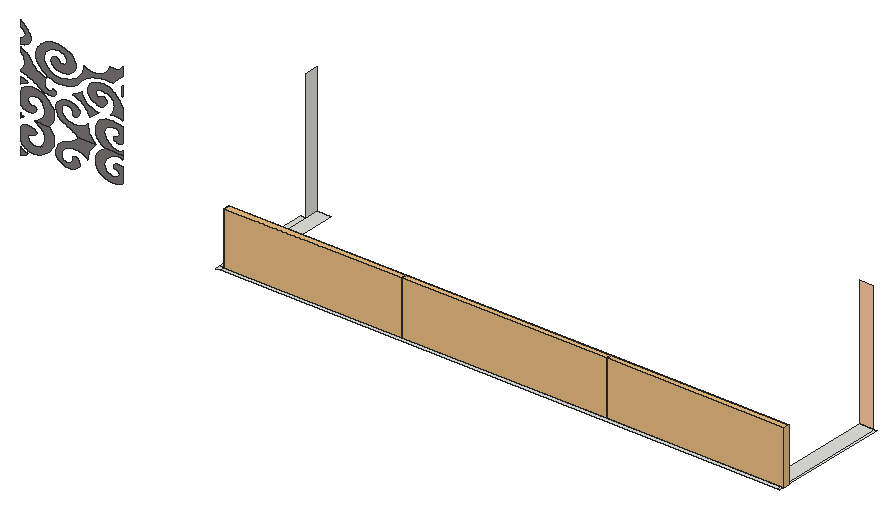
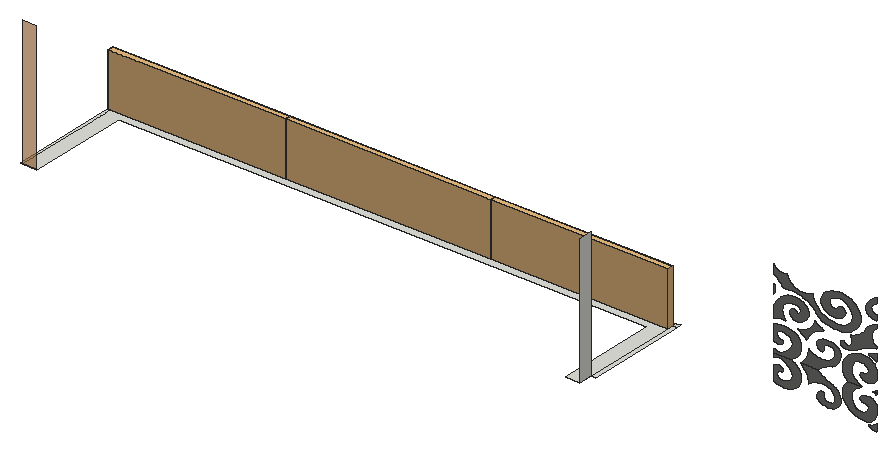
# SketchUp Ruby script. Lengths in inches.
U = 1.inch
M = Sketchup.active_model
def pt(a) = Geom::Point3d.new(a.map { |v| v * U })
def face(e, loops, mat)
  f = e.add_face(loops[0].map { |a| pt(a) })
  loops[1..].each { |l| e.add_face(l.map { |a| pt(a) }).erase! }
  f.material = f.back_material = mat if mat
  f
end
# faces: each face lists its corners as indices into pts; further lists are holes
def faces(e, pts, list, mat = nil) = list.each { |f| face(e, (f[0].is_a?(Array) ? f : [f]).map { |l| l.map { |i| pts[i] } }, mat) }
# xy, xz, yz: faces in a plane at the given z, y or x. An outline is a flat list of corners, or four numbers for a rectangle; further outlines are holes
def ring(l) = l.size == 4 ? [[l[0], l[1]], [l[2], l[1]], [l[2], l[3]], [l[0], l[3]]] : l.each_slice(2).to_a
def flat(e, list, mat, &to3) = list.each { |f| face(e, (f[0].is_a?(Array) ? f : [f]).map { |l| ring(l).map { |u, v| to3.(u, v) } }, mat) }
def xy(e, z, list, mat = nil) = flat(e, list, mat) { |x, y| [x, y, z] }
def xz(e, y, list, mat = nil) = flat(e, list, mat) { |x, z| [x, y, z] }
def yz(e, x, list, mat = nil) = flat(e, list, mat) { |y, z| [x, y, z] }
def lines(e, pts, list) = list.each { |a, b| e.add_line(pt(pts[a]), pt(pts[b])) }
# prism: a flat outline (further loops are holes) pulled along v
def prism(e, loops, v, mat = nil)
  f = face(e, loops, mat); d = Geom::Vector3d.new(v.map { |x| x * U })
  f.pushpull(f.normal.samedirection?(d) ? d.length : -d.length)
end
def box(e, o, s, mat = nil) = prism(e, [[o, [o[0] + s[0], o[1], o[2]], [o[0] + s[0], o[1] + s[1], o[2]], [o[0], o[1] + s[1], o[2]]]], [0, 0, s[2]], mat)
def at(x, y, z, deg = 0) = Geom::Transformation.translation(pt([x, y, z])) * Geom::Transformation.rotation(ORIGIN, Z_AXIS, deg.degrees)
def axes(o, x, y, z) = Geom::Transformation.new([*x, 0, *y, 0, *z, 0, *pt(o).to_a, 1])
def part(name) = M.definitions.add(name)
# library, detail: a bought-in or finely detailed component or shape, given as its bounding box
def library(name, o, s) = part(name).tap { |d| box(d.entities, o, s) }
def detail(e, o, s) = box(e.add_group.entities, o, s)
def put(e, d, t, mat = nil) = e.add_instance(d, t).tap { |i| i.material = mat if mat }
def group(e, t, mat = nil) = e.add_group.tap { |g| g.transformation = t; g.material = mat if mat }.entities
root = M.entities
M.materials.add("[0043_SaddleBrown]4").color = [124, 123, 122]
M.materials.add("[Granite Light Gray]").color = [149, 148, 144]
M.materials.add("[Wood Floor]").color = [224, 152, 88]
M.materials["[Wood Floor]"].alpha = 0.68
c1 = library("Glass Railing",[0,0,0],[139.5,4.76,42])
xy(root,293,[[1798.95,556.4375,1802.38,559.875],[1802.38,556.4375,2240.81,559.875],[2240.81,556.4375,2242.75,559.875],[1798.95,559.875,1802.38,640.11],[1802.38,559.875,2240.81,559.875,2240.81,651.03,2229.49,651.03,2229.49,571.2,1813.71,571.2,1813.71,651.03,1802.38,651.03],
  [2240.81,559.875,2242.75,651.03]])
xz(root,589.17,[[1618.6,295.77,1618.6,301,1618.96,300.64,1619.34,300.3,1619.76,299.98,1620.21,299.68,1620.6875,299.4,1621.1875,299.15,1621.71,298.92,1622.26,298.72,1622.82,298.54,1623.39,298.4,1623.98,298.28,1624.58,298.1875,1624.22,297.86,1623.82,297.54,1623.39,297.25,1622.9375,296.98,1622.46,296.74,1621.95,296.52,1621.43,296.32,1620.89,296.15,1620.33,296.02,1619.76,295.91,1619.18,295.82],[1656.57,299.46,1654.58,299.6,1652.66,300.03,1650.91,300.72,1649.39,301.66,1648.17,302.81,1647.3,304.1,1646.8,305.5,1646.66,306.54,1646.64,307.57,1646.74,308.61,1646.97,309.63,1647.32,310.64,1647.8,311.62,1648.39,312.57,1649.09,313.47,1649.9,314.33,1650.81,315.14,1651.81,315.88,1652.91,316.56,1654.06,316.875,1655.18,317.24,1656.28,317.65,1657.34,318.1,1658.37,318.59,1659.35,319.13,1660.3,319.7,1661.19,320.3125,1662.04,320.96,1662.84,321.64,1663.58,322.35,1664.27,323.09,1678.03,323.09,1677.05,322.2,1676.15,321.27,1675.33,320.31,1674.59,319.31,1673.93,318.28,1673.37,317.22,1672.9,316.14,1672.52,315.03,1672.24,313.92,1672.05,312.79,1671.96,311.66,1671.96,310.53,1671.38,311.07,1670.75,311.58,1670.07,312.0625,1669.34,312.51,1668.58,312.91,1667.77,313.28,1666.93,313.6,1666.0625,313.88,1665.17,314.11,1664.25,314.3,1663.32,314.44,1662.38,314.54,1660.75,314.5625,1659.14,314.41,1657.58,314.07,1656.12,313.56,1654.78,312.89,1653.61,312.07,1652.63,311.14,1651.87,310.1,1651.34,308.99,1651.06,307.84,1651.03,306.66,1651.27,305.5,1651.52,304.93,1651.91,304.41,1652.43,303.9375,1653.0625,303.54,1653.78,303.24,1654.5625,303.04,1655.38,302.93,1656.21,302.94,1657.03,303.06,1657.8,303.28,1658.51,303.6,1659.12,304,1659.28,304.24,1659.42,304.5,1659.55,304.75,1659.65,305.01,1659.73,305.28,1659.8,305.54,1659.84,305.8125,1659.86,306.08,1659.86,306.36,1659.84,306.625,1659.8,306.9,1659.74,307.16,1659.71,307.41,1659.73,307.66,1659.82,307.9,1659.96,308.13,1660.15,308.34,1660.39,308.52,1660.67,308.67,1660.98,308.78,1661.31,308.85,1661.65,308.875,1662,308.86,1662.33,308.8,1662.94,308.46,1663.49,308.07,1663.98,307.64,1664.4,307.17,1664.75,306.68,1665.02,306.15,1665.21,305.61,1665.32,305.0625,1665.34,304.51,1665.28,303.95,1665.14,303.41,1664.91,302.875,1663.71,301.72,1662.2,300.77,1660.46,300.06,1658.56,299.61],[1629.43,299.94,1627.86,299.97,1626.32,300.16,1624.83,300.52,1623.43,301.04,1622.16,301.7,1621.05,302.5,1620.12,303.41,1619.39,304.41,1618.88,305.48,1618.6,306.59,1618.6,314.54,1619.0625,315.41,1619.74,316.19,1620.61,316.875,1621.65,317.42,1622.81,317.82,1624.05,318.05,1625.33,318.11,1626.61,318,1627.83,317.71,1628.96,317.27,1629.94,316.67,1630.76,315.96,1631,315.64,1631.16,315.29,1631.23,314.93,1631.21,314.57,1631.09,314.22,1630.89,313.88,1630.61,313.58,1630.26,313.32,1629.85,313.11,1629.39,312.96,1628.91,312.86,1628.4,312.84,1627.74,312.8,1627.09,312.6875,1626.48,312.49,1625.93,312.23,1625.44,311.89,1625.05,311.51,1624.75,311.08,1624.56,310.62,1624.48,310.14,1624.52,309.66,1624.67,309.1875,1624.94,308.75,1625.32,307.98,1625.89,307.28,1626.64,306.67,1627.53,306.17,1628.53,305.8,1629.62,305.58,1630.74,305.5,1631.86,305.58,1632.95,305.81,1633.95,306.18,1635.37,307.48,1636.5,308.92,1637.31,310.46,1637.79,312.08,1637.91,313.73,1637.6875,315.38,1637.11,316.98,1636.21,318.5,1634.99,319.9,1633.49,321.15,1631.74,322.22,1629.79,323.09,1640.73,323.09,1642.56,321.23,1643.95,319.18,1644.89,317,1645.33,314.75,1645.27,312.47,1644.71,310.22,1643.67,308.07,1642.17,306.0625,1640.25,304.25,1637.96,302.68,1635.35,301.39,1632.49,300.42,1630.99,300.1],[1691.27,301.35,1688.56,301.57,1685.97,302.17,1683.6,303.12,1681.53,304.39,1679.84,305.93,1678.61,307.67,1677.88,309.5625,1677.68,311.52,1678.02,313.46,1678.1,314.46,1678.31,315.44,1678.63,316.41,1679.08,317.35,1679.65,318.26,1680.33,319.125,1681.12,319.94,1682.01,320.71,1682.99,321.41,1684.05,322.04,1685.19,322.6,1686.4,323.09,1698.99,323.09,1698.99,320.125,1698.69,320.4,1698.35,320.65,1697.96,320.87,1697.55,321.05,1697.11,321.2,1696.64,321.3,1696.17,321.37,1695.68,321.4,1695.19,321.38,1694.71,321.32,1694.25,321.23,1693.8,321.09,1692.72,320.67,1691.68,320.19,1690.7,319.66,1689.77,319.08,1688.9,318.45,1688.1,317.78,1687.37,317.07,1686.7,316.33,1686.12,315.55,1685.62,314.74,1685.19,313.91,1684.85,313.06,1684.66,312.23,1684.625,311.39,1684.77,310.55,1685.07,309.74,1685.54,308.97,1686.15,308.25,1686.9,307.61,1687.78,307.05,1688.76,306.59,1689.8125,306.24,1690.93,306,1692.09,305.875,1693.15,305.92,1694.17,306.14,1695.08,306.54,1695.83,307.09,1696.37,307.75,1696.67,308.49,1696.71,309.26,1696.49,310.01,1696.02,310.7,1695.33,311.28,1694.46,311.73,1693.47,312.01,1693.23,312,1692.98,312.01,1692.74,312.06,1692.52,312.13,1692.3125,312.23,1692.14,312.36,1691.99,312.5,1691.89,312.66,1691.82,312.83,1691.79,313.01,1691.81,313.18,1691.87,313.36,1692.15,313.84,1692.54,314.28,1693.03,314.67,1693.59,315,1694.22,315.25,1694.91,315.43,1695.62,315.53,1696.35,315.54,1697.0625,315.47,1697.76,315.3125,1698.4,315.08,1698.99,314.77,1698.99,302.99,1696.58,302.08,1693.98,301.53],[1618.6,321.36,1618.6,323.09,1621,323.09,1620.68,323.07,1620.38,323.03,1620.08,322.96,1619.8,322.86,1619.54,322.73,1619.3,322.58,1619.1,322.41,1618.92,322.22,1618.78,322.02,1618.68,321.81,1618.62,321.59],
  [1618.6,323.09,1621,323.09,1620.68,323.1,1620.38,323.15,1620.08,323.22,1619.8,323.32,1619.54,323.45,1619.3,323.59,1619.1,323.76,1618.92,323.95,1618.78,324.16,1618.68,324.37,1618.62,324.59,1618.6,324.82],[1629.79,323.09,1640.73,323.09,1642.56,324.95,1643.95,326.99,1644.89,329.17,1645.33,331.43,1645.27,333.71,1644.71,335.95,1643.67,338.11,1642.17,340.11,1640.25,341.93,1637.96,343.5,1635.35,344.78,1632.49,345.76,1630.99,346.08,1629.43,346.23,1627.86,346.21,1626.32,346.02,1624.83,345.66,1623.43,345.14,1622.16,344.47,1621.05,343.68,1620.12,342.77,1619.39,341.77,1618.88,340.7,1618.6,339.58,1618.6,331.63,1619.0625,330.77,1619.74,329.98,1620.61,329.3,1621.65,328.75,1622.81,328.36,1624.05,328.12,1625.33,328.0625,1626.61,328.18,1627.83,328.46,1628.96,328.91,1629.94,329.5,1630.76,330.22,1631,330.54,1631.16,330.88,1631.23,331.24,1631.21,331.61,1631.09,331.96,1630.89,332.29,1630.61,332.6,1630.26,332.86,1629.85,333.07,1629.39,333.22,1628.91,333.3125,1628.4,333.34,1627.74,333.375,1627.09,333.49,1626.48,333.68,1625.93,333.95,1625.44,334.28,1625.05,334.67,1624.75,335.1,1624.56,335.5625,1624.48,336.04,1624.52,336.52,1624.67,336.99,1624.94,337.43,1625.32,338.2,1625.89,338.9,1626.64,339.51,1627.53,340,1628.53,340.375,1629.62,340.6,1630.74,340.68,1631.86,340.6,1632.95,340.37,1633.95,340,1635.37,338.7,1636.5,337.26,1637.31,335.71,1637.79,334.1,1637.91,332.44,1637.6875,330.8,1637.11,329.2,1636.21,327.68,1634.99,326.28,1633.49,325.02,1631.74,323.95],[1664.27,323.09,1678.03,323.09,1677.05,323.97,1676.15,324.9,1675.33,325.87,1674.59,326.87,1673.93,327.9,1673.37,328.96,1672.9,330.04,1672.52,331.14,1672.24,332.26,1672.05,333.38,1671.96,334.51,1671.96,335.65,1671.38,335.11,1670.75,334.59,1670.07,334.11,1669.34,333.67,1668.58,333.27,1667.77,332.9,1666.93,332.58,1666.0625,332.3,1665.17,332.0625,1664.25,331.875,1663.32,331.73,1662.38,331.64,1660.75,331.61,1659.14,331.77,1657.58,332.11,1656.12,332.62,1654.78,333.29,1653.61,334.1,1652.63,335.04,1651.87,336.08,1651.34,337.18,1651.06,338.34,1651.03,339.51,1651.27,340.67,1651.52,341.24,1651.91,341.77,1652.43,342.24,1653.0625,342.63,1653.78,342.9375,1654.5625,343.14,1655.38,343.24,1656.21,343.23,1657.03,343.12,1657.8,342.9,1658.51,342.58,1659.12,342.18,1659.28,341.93,1659.42,341.68,1659.55,341.42,1659.65,341.16,1659.73,340.9,1659.8,340.63,1659.84,340.36,1659.86,340.09,1659.86,339.82,1659.84,339.55,1659.8,339.28,1659.74,339.01,1659.71,338.76,1659.73,338.52,1659.82,338.27,1659.96,338.05,1660.15,337.84,1660.39,337.66,1660.67,337.51,1660.98,337.4,1661.31,337.33,1661.65,337.3,1662,337.32,1662.33,337.37,1662.94,337.72,1663.49,338.11,1663.98,338.54,1664.4,339,1664.75,339.5,1665.02,340.02,1665.21,340.5625,1665.32,341.11,1665.34,341.67,1665.28,342.22,1665.14,342.77,1664.91,343.3,1663.71,344.45,1662.2,345.41,1660.46,346.12,1658.56,346.5625,1656.57,346.72,1654.58,346.58,1652.66,346.15,1650.91,345.45,1649.39,344.51,1648.17,343.37,1647.3,342.07,1646.8,340.67,1646.66,339.64,1646.64,338.6,1646.74,337.57,1646.97,336.54,1647.32,335.54,1647.8,334.56,1648.39,333.61,1649.09,332.7,1649.9,331.84,1650.81,331.04,1651.81,330.3,1652.91,329.62,1654.06,329.3,1655.18,328.9375,1656.28,328.53,1657.34,328.08,1658.37,327.58,1659.35,327.05,1660.3,326.47,1661.19,325.86,1662.04,325.22,1662.84,324.54,1663.58,323.83],[1686.4,323.09,1698.99,323.09,1698.99,326.05,1698.69,325.77,1698.35,325.53,1697.96,325.31,1697.55,325.125,1697.11,324.98,1696.64,324.87,1696.17,324.8,1695.68,324.78,1695.19,324.79,1694.71,324.85,1694.25,324.95,1693.8,325.09,1692.72,325.51,1691.68,325.99,1690.7,326.52,1689.77,327.1,1688.9,327.72,1688.1,328.39,1687.37,329.1,1686.7,329.85,1686.12,330.625,1685.62,331.43,1685.19,332.27,1684.85,333.12,1684.66,333.95,1684.625,334.79,1684.77,335.62,1685.07,336.44,1685.54,337.21,1686.15,337.92,1686.9,338.57,1687.78,339.125,1688.76,339.58,1689.8125,339.9375,1690.93,340.18,1692.09,340.3,1693.15,340.26,1694.17,340.03,1695.08,339.64,1695.83,339.09,1696.37,338.43,1696.67,337.6875,1696.71,336.92,1696.49,336.17,1696.02,335.48,1695.33,334.89,1694.46,334.45,1693.47,334.17,1693.23,334.18,1692.98,334.17,1692.74,334.12,1692.52,334.05,1692.3125,333.95,1692.14,333.82,1691.99,333.68,1691.89,333.52,1691.82,333.35,1691.79,333.17,1691.81,332.99,1691.87,332.82,1692.15,332.34,1692.54,331.9,1693.03,331.51,1693.59,331.18,1694.22,330.92,1694.91,330.74,1695.62,330.65,1696.35,330.64,1697.0625,330.71,1697.76,330.86,1698.4,331.1,1698.99,331.41,1698.99,343.1875,1696.58,344.1,1693.98,344.65,1691.27,344.82,1688.56,344.61,1685.97,344.01,1683.6,343.06,1681.53,341.79,1679.84,340.25,1678.61,338.5,1677.88,336.61,1677.68,334.66,1678.02,332.71,1678.1,331.72,1678.31,330.74,1678.63,329.77,1679.08,328.83,1679.65,327.92,1680.33,327.05,1681.12,326.23,1682.01,325.47,1682.99,324.77,1684.05,324.13,1685.19,323.57],[1673.16,341.21,1673.69,341.68,1674.23,342.15,1674.78,342.61,1675.34,343.0625,1675.91,343.51,1676.5,343.95,1677.09,344.38,1677.6875,344.81,1678.3,345.23,1678.92,345.64,1679.55,346.04,1680.1875,346.4375,1678.52,346.72,1676.9,347.12,1675.36,347.65,1673.9,348.29,1672.55,349.05,1671.3125,349.9,1670.21,350.85,1669.26,351.87,1668.47,352.97,1667.84,354.11,1667.39,355.3,1667.12,356.52,1666.57,356.14,1666.01,355.77,1665.44,355.4,1664.87,355.04,1664.28,354.69,1663.6875,354.35,1663.09,354.02,1662.47,353.6875,1661.86,353.37,1660.6,352.75,1659.95,352.46,1661.56,351.92,1663.1,351.3,1664.5625,350.58,1665.95,349.79,1667.24,348.92,1668.4375,347.98,1669.52,346.98,1670.5,345.91,1671.36,344.8,1672.09,343.64,1672.69,342.4375],
  [1618.6,345.18,1618.96,345.53,1619.34,345.875,1619.76,346.2,1620.21,346.5,1620.6875,346.77,1621.1875,347.03,1621.71,347.26,1622.26,347.46,1622.82,347.63,1623.39,347.78,1623.98,347.9,1624.58,347.99,1624.22,348.32,1623.82,348.63,1623.39,348.93,1622.9375,349.19,1622.46,349.44,1621.95,349.66,1621.43,349.85,1620.89,350.02,1620.33,350.16,1619.76,350.27,1619.18,350.35,1618.6,350.4],[1642.25,345.8,1643.26,345.82,1644.08,345.91,1644.84,346.14,1645.52,346.49,1646.0625,346.93,1646.46,347.45,1646.68,348.03,1646.72,348.625,1646.57,349.21,1646.24,349.76,1645.75,350.24,1645.125,350.625,1644.39,350.9,1644.28,350.3,1643.96,349.75,1643.46,349.27,1642.79,348.9,1642.02,348.67,1641.19,348.59,1640.36,348.67,1639.59,348.9,1638.93,349.27,1638.42,349.75,1638.1,350.3,1637.99,350.9,1637.95,351.375,1637.92,351.85,1637.91,352.33,1637.92,352.8,1637.95,353.28,1637.99,353.75,1638.05,354.22,1638.13,354.7,1638.23,355.17,1638.35,355.63,1638.48,356.1,1638.63,356.5625,1637.17,356.99,1635.75,357.49,1634.4,358.08,1633.12,358.74,1631.91,359.47,1630.79,360.27,1629.76,361.14,1628.83,362.05,1628,363.02,1627.28,364.03,1626.68,365.09,1626.19,366.17,1625.67,366.67,1625.12,367.16,1624.55,367.64,1623.97,368.1,1623.36,368.55,1622.73,368.99,1622.09,369.41,1621.42,369.82,1620.74,370.21,1620.04,370.59,1619.33,370.95,1618.6,371.29,1618.6,368.08,1619.62,367.17,1620.48,366.18,1621.16,365.12,1621.65,364.01,1621.95,362.86,1622.05,361.69,1621.95,360.52,1621.65,359.375,1621.16,358.26,1620.48,357.2,1619.62,356.21,1618.6,355.3,1618.6,354.25,1619.89,354.05,1621.16,353.81,1622.41,353.53,1623.64,353.19,1624.85,352.8125,1626.02,352.39,1627.16,351.92,1628.27,351.4,1629.33,350.85,1630.36,350.26,1631.34,349.63,1632.28,348.96,1633,348.45,1633.78,347.98,1634.6,347.55,1635.47,347.16,1636.36,346.82,1637.29,346.53,1638.25,346.28,1639.23,346.08,1640.23,345.9375,1641.23,345.85],[1698.99,347.78,1698.99,356.71,1698.625,357.36,1698.25,358,1697.85,358.64,1697.4375,359.27,1697.01,359.9,1696.57,360.52,1696.11,361.13,1695.64,361.74,1695.16,362.35,1694.65,362.95,1694.14,363.54,1693.61,364.12,1692.75,364.94,1691.77,365.6875,1690.67,366.34,1689.48,366.9,1688.2,367.36,1686.86,367.71,1685.48,367.94,1684.0625,368.0625,1682.64,368.0625,1681.22,367.94,1679.84,367.71,1678.5,367.36,1676.5625,366.59,1674.87,365.57,1673.48,364.33,1672.45,362.92,1671.82,361.39,1671.6,359.81,1671.82,358.23,1672.45,356.7,1673.48,355.29,1674.87,354.05,1676.5625,353.03,1678.5,352.26,1679.14,351.99,1679.83,351.8,1680.56,351.6875,1681.3,351.66,1682.04,351.71,1682.76,351.86,1683.43,352.08,1684.05,352.37,1684.6,352.73,1685.0625,353.15,1685.43,353.62,1685.68,354.12,1686.05,354.57,1686.32,355.05,1686.5,355.55,1686.58,356.0625,1686.55,356.58,1686.43,357.09,1686.2,357.59,1685.88,358.05,1685.48,358.48,1684.99,358.86,1684.4375,359.19,1683.82,359.46,1683.47,359.32,1683.13,359.17,1682.8,359,1682.49,358.82,1682.2,358.62,1681.93,358.41,1681.68,358.18,1681.45,357.94,1681.25,357.69,1681.07,357.43,1680.91,357.17,1680.79,356.89,1680.02,357.23,1679.35,357.65,1678.81,358.17,1678.41,358.74,1678.16,359.36,1678.08,360,1678.16,360.64,1678.41,361.26,1678.81,361.84,1679.35,362.35,1680.02,362.78,1680.79,363.11,1681.72,363.13,1682.65,363.11,1683.58,363.03,1684.5,362.91,1685.4,362.73,1686.28,362.51,1687.14,362.24,1687.96,361.93,1688.75,361.57,1689.51,361.17,1690.22,360.73,1690.88,360.26,1691.46,359.34,1691.93,358.39,1692.28,357.41,1692.5,356.41,1692.6,355.41,1692.57,354.4,1692.42,353.39,1692.14,352.4,1691.74,351.4375,1691.22,350.5,1690.58,349.6,1689.84,348.74,1690.6,348.93,1691.38,349.07,1692.18,349.17,1692.98,349.21,1693.79,349.2,1694.59,349.14,1695.38,349.03,1696.16,348.875,1696.91,348.67,1697.64,348.42,1698.34,348.12],[1649.27,356.35,1652.43,356.47,1655.52,356.98,1658.4375,357.86,1661.11,359.07,1663.46,360.6,1665.42,362.39,1665.96,363.14,1666.55,363.86,1667.18,364.5625,1667.87,365.25,1668.59,365.9,1669.36,366.53,1670.17,367.14,1671.01,367.72,1671.9,368.26,1672.82,368.78,1673.77,369.26,1674.75,369.72,1676.05,370.16,1677.39,370.56,1678.75,370.9,1680.14,371.18,1681.54,371.41,1682.96,371.59,1684.4,371.7,1685.84,371.76,1687.28,371.77,1688.72,371.71,1690.15,371.6,1691.58,371.43,1692.13,372.07,1692.7,372.71,1693.28,373.34,1693.87,373.96,1694.47,374.58,1695.08,375.19,1695.71,375.8,1696.34,376.4,1696.99,376.99,1697.65,377.58,1698.3125,378.16,1698.99,378.74,1698.99,385.48,1698.625,384.78,1698.125,384.13,1697.51,383.54,1696.78,383.01,1695.95,382.5625,1695.05,382.2,1694.09,381.9375,1693.08,381.77,1692.05,381.71,1691.02,381.75,1690.01,381.9,1689.03,382.14,1688.59,380.54,1687.78,379.02,1686.61,377.62,1685.13,376.38,1683.38,375.35,1681.41,374.54,1679.28,373.99,1677.05,373.7,1674.79,373.7,1672.55,373.98,1670.42,374.52,1668.45,375.32,1668.38,373.3,1667.92,371.31,1667.05,369.39,1665.8125,367.57,1664.22,365.91,1662.31,364.43,1660.12,363.17,1657.7,362.14,1655.1,361.39,1652.38,360.91,1649.59,360.72,1646.79,360.82,1644.34,361.55,1642.12,362.6,1640.23,363.94,1638.74,365.52,1637.69,367.27,1637.14,369.14,1637.09,371.05,1637.5625,372.94,1638.53,374.72,1639.95,376.33,1641.77,377.71,1643.9375,378.82,1645.33,379.26,1646.82,379.49,1648.35,379.5,1649.84,379.28,1651.24,378.85,1652.5,378.22,1653.54,377.42,1654.34,376.48,1654.86,375.45,1655.07,374.36,1654.97,373.26,1654.56,372.2,1654.29,371.81,1653.91,371.47,1653.45,371.19,1652.91,370.98,1652.34,370.85,1651.73,370.81,1651.13,370.85,1650.55,370.98,1650.02,371.19,1649.55,371.47,1649.18,371.81,1648.9,372.2,1648.76,372.43,1648.6,372.65,1648.41,372.85,1648.2,373.05,1647.97,373.23,1647.72,373.4,1647.46,373.55,1647.17,373.6875,1646.87,373.81,1646.56,373.91,1646.24,373.99,1645.91,374.05,1645.33,373.81,1644.79,373.51,1644.31,373.17,1643.89,372.79,1643.54,372.37,1643.26,371.93,1643.06,371.47,1642.9375,370.99,1642.9,370.5,1642.94,370.02,1643.07,369.54,1643.27,369.08,1643.66,368.45,1644.14,367.87,1644.71,367.32,1645.35,366.82,1646.07,366.37,1646.84,365.98,1647.67,365.65,1648.55,365.39,1649.45,365.2,1650.38,365.08,1651.33,365.03,1652.27,365.05,1653.77,365.22,1655.21,365.53,1656.59,365.98,1657.87,366.56,1659.04,367.25,1660.06,368.05,1660.93,368.95,1661.62,369.91,1662.13,370.9375,1662.45,372,1662.5625,373.09,1662.48,374.18,1661.87,375.81,1660.95,377.37,1659.73,378.8125,1658.24,380.12,1656.5,381.26,1654.5625,382.21,1652.45,382.95,1650.22,383.47,1647.91,383.76,1645.5625,383.8,1643.23,383.61,1640.96,383.18,1638.77,382.09,1636.78,380.8125,1635.05,379.36,1633.59,377.75,1632.43,376.03,1631.59,374.21,1631.09,372.32,1630.92,370.41,1631.1,368.5,1631.63,366.62,1632.49,364.8,1633.66,363.08,1635.47,361.21,1637.69,359.58,1640.25,358.25,1643.1,357.25,1646.13,356.61],[1698.99,364.66,1698.99,371.94,1698.77,371.35,1698.58,370.75,1698.4375,370.14,1698.33,369.53,1698.27,368.92,1698.25,368.3,1698.27,367.69,1698.33,367.07,1698.4375,366.46,1698.58,365.85,1698.77,365.25],
  [1618.6,373.83,1619.85,373.9,1621.07,374.11,1622.23,374.45,1623.31,374.91,1624.27,375.49,1625.11,376.16,1625.79,376.92,1626.3125,377.74,1626.65,378.61,1626.8,379.51,1626.76,380.41,1626.54,381.3,1626.1875,382.16,1625.78,383.01,1625.3,383.84,1624.77,384.65,1624.18,385.45,1623.54,386.22,1622.84,386.96,1622.09,387.68,1621.29,388.36,1620.4375,389.02,1619.54,389.64,1618.6,390.23,1618.6,385.49,1619.68,385.16,1620.65,384.67,1621.45,384.05,1622.05,383.32,1622.42,382.52,1622.54,381.67,1622.42,380.83,1622.05,380.02,1621.45,379.29,1620.65,378.67,1619.68,378.18,1618.6,377.85]],"[0043_SaddleBrown]4")
xz(root,651.03,[[2229.49,293,2240.81,394.4375]],"[Wood Floor]")
yz(root,1802.38,[[640.11,293,651.03,394.4375]])
p = [[1633.95,589.17,306.18],[1634.84,589.17,306.68],[1635.58,589.17,307.29],[1633.95,589.17,340],[1634.84,589.17,339.5],[1635.58,589.17,338.89]]
lines(root,p,[[0,1],[1,2],[3,4],[4,5]])
put(root,c1,at(1802.38,559.875,293))
put(root,c1,axes([1941.88,559.875,293],[1.15726,0,0],[0,1,0],[0,0,1]),"[Granite Light Gray]")
put(root,c1,at(2103.32,559.875,293))
